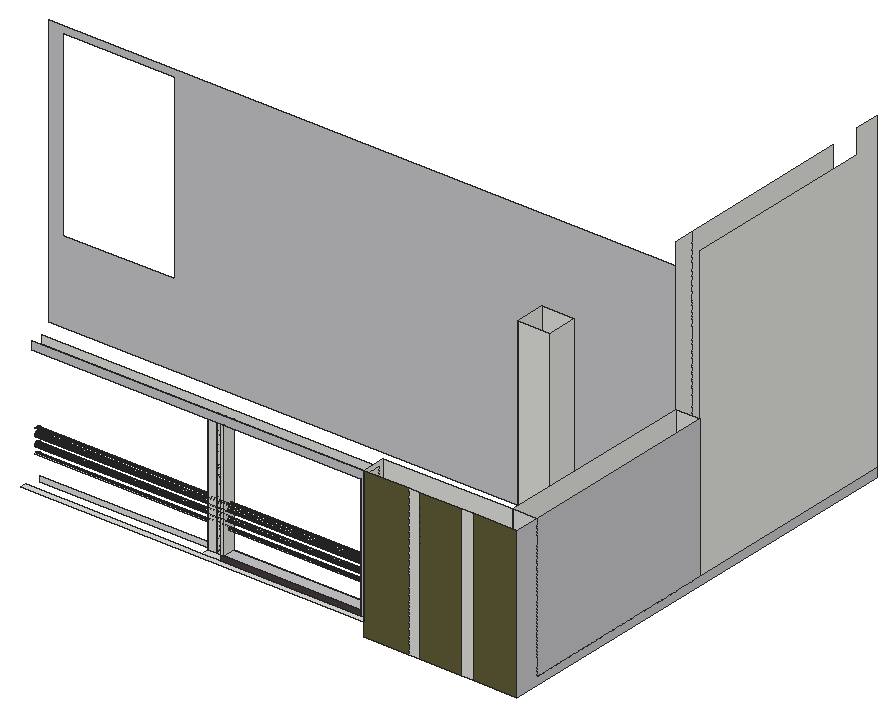
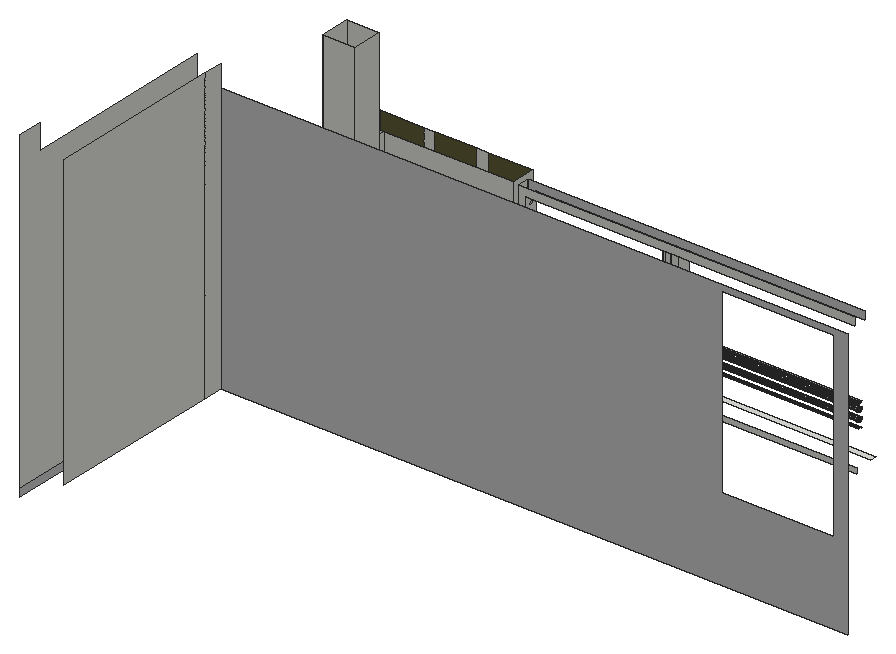
# SketchUp Ruby script. Lengths in inches.
U = 1.inch
M = Sketchup.active_model
def pt(a) = Geom::Point3d.new(a.map { |v| v * U })
def face(e, loops, mat)
  f = e.add_face(loops[0].map { |a| pt(a) })
  loops[1..].each { |l| e.add_face(l.map { |a| pt(a) }).erase! }
  f.material = f.back_material = mat if mat
  f
end
# faces: each face lists its corners as indices into pts; further lists are holes
def faces(e, pts, list, mat = nil) = list.each { |f| face(e, (f[0].is_a?(Array) ? f : [f]).map { |l| l.map { |i| pts[i] } }, mat) }
# xy, xz, yz: faces in a plane at the given z, y or x. An outline is a flat list of corners, or four numbers for a rectangle; further outlines are holes
def ring(l) = l.size == 4 ? [[l[0], l[1]], [l[2], l[1]], [l[2], l[3]], [l[0], l[3]]] : l.each_slice(2).to_a
def flat(e, list, mat, &to3) = list.each { |f| face(e, (f[0].is_a?(Array) ? f : [f]).map { |l| ring(l).map { |u, v| to3.(u, v) } }, mat) }
def xy(e, z, list, mat = nil) = flat(e, list, mat) { |x, y| [x, y, z] }
def xz(e, y, list, mat = nil) = flat(e, list, mat) { |x, z| [x, y, z] }
def yz(e, x, list, mat = nil) = flat(e, list, mat) { |y, z| [x, y, z] }
def lines(e, pts, list) = list.each { |a, b| e.add_line(pt(pts[a]), pt(pts[b])) }
# prism: a flat outline (further loops are holes) pulled along v
def prism(e, loops, v, mat = nil)
  f = face(e, loops, mat); d = Geom::Vector3d.new(v.map { |x| x * U })
  f.pushpull(f.normal.samedirection?(d) ? d.length : -d.length)
end
def box(e, o, s, mat = nil) = prism(e, [[o, [o[0] + s[0], o[1], o[2]], [o[0] + s[0], o[1] + s[1], o[2]], [o[0], o[1] + s[1], o[2]]]], [0, 0, s[2]], mat)
def at(x, y, z, deg = 0) = Geom::Transformation.translation(pt([x, y, z])) * Geom::Transformation.rotation(ORIGIN, Z_AXIS, deg.degrees)
def axes(o, x, y, z) = Geom::Transformation.new([*x, 0, *y, 0, *z, 0, *pt(o).to_a, 1])
def part(name) = M.definitions.add(name)
# library, detail: a bought-in or finely detailed component or shape, given as its bounding box
def library(name, o, s) = part(name).tap { |d| box(d.entities, o, s) }
def detail(e, o, s) = box(e.add_group.entities, o, s)
def put(e, d, t, mat = nil) = e.add_instance(d, t).tap { |i| i.material = mat if mat }
def group(e, t, mat = nil) = e.add_group.tap { |g| g.transformation = t; g.material = mat if mat }.entities
root = M.entities
M.materials.add("[0057_DarkKhaki]").color = [96, 93, 54]
M.materials.add("[Asphalt New]").color = [67, 60, 62]
M.materials.add("[Polished Concrete New]").color = [200, 200, 203]
M.materials.add("[Polished Concrete Old]").color = [229, 229, 229]
xy(root,9,[[1072.84,249.9,1099.23,472.99],[1027.11,314.12,1062.63,346.6]])
xy(root,14.9375,[[555.05,223.5,931.07,223.5,931.07,230.1,922.51,230.1,922.51,230.11,768.81,230.26,748.36,230.28,727.92,230.3,555.05,230.47],[922.51,230.1,922.51,230.11,931.07,230.1],[931.07,230.1,931.07,243.6875,922.51,243.6875,922.51,230.11],[922.51,230.11,768.81,230.26,768.82,243.84,931.07,243.6875,922.51,243.6875],[768.81,230.26,748.36,230.28,748.38,243.86,768.82,243.84]])
xy(root,21,[[754.67,230.27,754.67,243.86,764.33,243.85,764.33,230.27]])
xy(root,21,[[922.51,230.11,922.51,243.6875,931.07,243.6875,772.74,243.84,772.74,230.26]],"[Polished Concrete New]")
xz(root,223.5,[[980.52,0,992.48,163.5625],[1038.1875,0,1050.15,163.5625]])
xz(root,223.5,[[931.03,0,980.52,0,980.52,163.5625,931.07,163.5625,931.07,14.9375,931.03,14.9375],[992.48,0,1038.1875,163.5625],[1050.15,0,1099.23,163.5625]],"[0057_DarkKhaki]")
xz(root,230.1,[[922.51,14.9375,931.07,14.9375,931.07,158,562.43,158,562.43,149.47,922.51,149.47]],"[Polished Concrete New]")
xz(root,230.26,[[768.81,21,772.74,149.47],[768.81,21,772.74,149.47]])
xz(root,230.27,[[754.67,21,764.33,149.47]])
xz(root,243.6875,[[922.51,14.9375,931.07,21],[922.51,21,922.51,149.47,562.43,149.47,562.43,158.26,931.07,158.26,931.07,21]])
xz(root,249.9,[[555.05,9,931.07,14.9375],[931.07,9,1072.84,163.5625],[1072.84,9,1099.23,163.5625]])
xz(root,314.12,[[1027.11,9,1062.63,304.3125]])
xz(root,346.6,[[1027.11,9,1062.63,304.3125]])
xz(root,472.99,[[1072.84,9,1099.23,163.5625]])
xz(root,472.99,[[[386.67,9,1072.84,304.3125],[402.52,98.87,525.08,297.18]]],"[Polished Concrete New]")
yz(root,754.67,[[230.27,21,243.86,149.47]])
yz(root,764.33,[[230.27,21,243.85,149.47]])
yz(root,772.74,[[230.26,21,243.84,149.47]])
yz(root,922.51,[[[230.1,14.9375,230.1,149.47,243.6875,149.47,243.6875,21,230.11,21,230.11,14.9375],[236.62,77.51,237.7,77.65,238.71,78.07,239.58,78.74,240.24,79.6,240.66,80.61,240.81,81.7,240.66,82.78,240.24,83.79,239.58,84.66,238.71,85.32,237.7,85.74,236.62,85.89,235.53,85.74,234.52,85.32,233.66,84.66,232.99,83.79,232.57,82.78,232.43,81.7,232.57,80.61,232.99,79.6,233.66,78.74,234.52,78.07,235.53,77.65],[236.71,138.15,237.35,138.24,237.93,138.48,238.4375,138.87,238.83,139.375,239.07,139.96,239.15,140.59,239.07,141.22,238.83,141.8125,238.4375,142.32,237.93,142.7,237.35,142.95,236.71,143.03,236.08,142.95,235.5,142.7,234.99,142.32,234.6,141.8125,234.36,141.22,234.28,140.59,234.36,139.96,234.6,139.375,234.99,138.87,235.5,138.48,236.08,138.24],[236.71,89.28,237.35,89.36,237.93,89.61,238.4375,89.99,238.83,90.5,239.07,91.09,239.15,91.72,239.07,92.35,238.83,92.9375,238.4375,93.44,237.93,93.83,237.35,94.07,236.71,94.15,236.08,94.07,235.5,93.83,234.99,93.44,234.6,92.9375,234.36,92.35,234.28,91.72,234.36,91.09,234.6,90.5,234.99,89.99,235.5,89.61,236.08,89.36],[236.71,129.34,237.35,129.43,237.93,129.67,238.4375,130.06,238.83,130.5625,239.07,131.15,239.15,131.78,239.07,132.41,238.83,133,238.4375,133.5,237.93,133.89,237.35,134.13,236.71,134.22,236.08,134.13,235.5,133.89,234.99,133.5,234.6,133,234.36,132.41,234.28,131.78,234.36,131.15,234.6,130.5625,234.99,130.06,235.5,129.67,236.08,129.43],[236.71,98.28,237.35,98.36,237.93,98.61,238.4375,98.99,238.83,99.5,239.07,100.09,239.15,100.72,239.07,101.35,238.83,101.9375,238.4375,102.44,237.93,102.83,237.35,103.07,236.71,103.15,236.08,103.07,235.5,102.83,234.99,102.44,234.6,101.9375,234.36,101.35,234.28,100.72,234.36,100.09,234.6,99.5,234.99,98.99,235.5,98.61,236.08,98.36],[236.71,118.53,237.35,118.61,237.93,118.86,238.4375,119.24,238.83,119.75,239.07,120.34,239.15,120.97,239.07,121.6,238.83,122.1875,238.4375,122.69,237.93,123.08,237.35,123.32,236.71,123.4,236.08,123.32,235.5,123.08,234.99,122.69,234.6,122.1875,234.36,121.6,234.28,120.97,234.36,120.34,234.6,119.75,234.99,119.24,235.5,118.86,236.08,118.61],[236.71,108.15,237.35,108.24,237.93,108.48,238.4375,108.87,238.83,109.375,239.07,109.96,239.15,110.59,239.07,111.22,238.83,111.8125,238.4375,112.32,237.93,112.7,237.35,112.95,236.71,113.03,236.08,112.95,235.5,112.7,234.99,112.32,234.6,111.8125,234.36,111.22,234.28,110.59,234.36,109.96,234.6,109.375,234.99,108.87,235.5,108.48,236.08,108.24],[236.71,23.9,237.35,23.99,237.93,24.23,238.4375,24.62,238.83,25.125,239.07,25.71,239.15,26.34,239.07,26.97,238.83,27.5625,238.4375,28.07,237.93,28.45,237.35,28.7,236.71,28.78,236.08,28.7,235.5,28.45,234.99,28.07,234.6,27.5625,234.36,26.97,234.28,26.34,234.36,25.71,234.6,25.125,234.99,24.62,235.5,24.23,236.08,23.99],[236.71,70.22,237.35,70.3,237.93,70.54,238.4375,70.93,238.83,71.4375,239.07,72.02,239.15,72.65,239.07,73.29,238.83,73.875,238.4375,74.38,237.93,74.77,237.35,75.01,236.71,75.09,236.08,75.01,235.5,74.77,234.99,74.38,234.6,73.875,234.36,73.29,234.28,72.65,234.36,72.02,234.6,71.4375,234.99,70.93,235.5,70.54,236.08,70.3],[236.71,33.4,237.35,33.49,237.93,33.73,238.4375,34.12,238.83,34.625,239.07,35.21,239.15,35.84,239.07,36.47,238.83,37.0625,238.4375,37.57,237.93,37.95,237.35,38.2,236.71,38.28,236.08,38.2,235.5,37.95,234.99,37.57,234.6,37.0625,234.36,36.47,234.28,35.84,234.36,35.21,234.6,34.625,234.99,34.12,235.5,33.73,236.08,33.49],[236.71,61.84,237.35,61.93,237.93,62.17,238.4375,62.56,238.83,63.0625,239.07,63.65,239.15,64.28,239.07,64.91,238.83,65.5,238.4375,66,237.93,66.39,237.35,66.63,236.71,66.72,236.08,66.63,235.5,66.39,234.99,66,234.6,65.5,234.36,64.91,234.28,64.28,234.36,63.65,234.6,63.0625,234.99,62.56,235.5,62.17,236.08,61.93],[236.71,41.84,237.35,41.93,237.93,42.17,238.4375,42.56,238.83,43.0625,239.07,43.65,239.15,44.28,239.07,44.91,238.83,45.5,238.4375,46,237.93,46.39,237.35,46.63,236.71,46.72,236.08,46.63,235.5,46.39,234.99,46,234.6,45.5,234.36,44.91,234.28,44.28,234.36,43.65,234.6,43.0625,234.99,42.56,235.5,42.17,236.08,41.93],[236.71,52.03,237.35,52.11,237.93,52.36,238.4375,52.74,238.83,53.25,239.07,53.84,239.15,54.47,239.07,55.1,238.83,55.6875,238.4375,56.19,237.93,56.58,237.35,56.82,236.71,56.9,236.08,56.82,235.5,56.58,234.99,56.19,234.6,55.6875,234.36,55.1,234.28,54.47,234.36,53.84,234.6,53.25,234.99,52.74,235.5,52.36,236.08,52.11]],[230.11,14.9375,243.6875,21],[236.71,23.9,237.35,23.99,237.93,24.23,238.4375,24.62,238.83,25.125,239.07,25.71,239.15,26.34,239.07,26.97,238.83,27.5625,238.4375,28.07,237.93,28.45,237.35,28.7,236.71,28.78,236.08,28.7,235.5,28.45,234.99,28.07,234.6,27.5625,234.36,26.97,234.28,26.34,234.36,25.71,234.6,25.125,234.99,24.62,235.5,24.23,236.08,23.99],[236.71,33.4,237.35,33.49,237.93,33.73,238.4375,34.12,238.83,34.625,239.07,35.21,239.15,35.84,239.07,36.47,238.83,37.0625,238.4375,37.57,237.93,37.95,237.35,38.2,236.71,38.28,236.08,38.2,235.5,37.95,234.99,37.57,234.6,37.0625,234.36,36.47,234.28,35.84,234.36,35.21,234.6,34.625,234.99,34.12,235.5,33.73,236.08,33.49],[236.71,41.84,237.35,41.93,237.93,42.17,238.4375,42.56,238.83,43.0625,239.07,43.65,239.15,44.28,239.07,44.91,238.83,45.5,238.4375,46,237.93,46.39,237.35,46.63,236.71,46.72,236.08,46.63,235.5,46.39,234.99,46,234.6,45.5,234.36,44.91,234.28,44.28,234.36,43.65,234.6,43.0625,234.99,42.56,235.5,42.17,236.08,41.93],
  [236.71,52.03,237.35,52.11,237.93,52.36,238.4375,52.74,238.83,53.25,239.07,53.84,239.15,54.47,239.07,55.1,238.83,55.6875,238.4375,56.19,237.93,56.58,237.35,56.82,236.71,56.9,236.08,56.82,235.5,56.58,234.99,56.19,234.6,55.6875,234.36,55.1,234.28,54.47,234.36,53.84,234.6,53.25,234.99,52.74,235.5,52.36,236.08,52.11],[236.71,61.84,237.35,61.93,237.93,62.17,238.4375,62.56,238.83,63.0625,239.07,63.65,239.15,64.28,239.07,64.91,238.83,65.5,238.4375,66,237.93,66.39,237.35,66.63,236.71,66.72,236.08,66.63,235.5,66.39,234.99,66,234.6,65.5,234.36,64.91,234.28,64.28,234.36,63.65,234.6,63.0625,234.99,62.56,235.5,62.17,236.08,61.93],[236.71,70.22,237.35,70.3,237.93,70.54,238.4375,70.93,238.83,71.4375,239.07,72.02,239.15,72.65,239.07,73.29,238.83,73.875,238.4375,74.38,237.93,74.77,237.35,75.01,236.71,75.09,236.08,75.01,235.5,74.77,234.99,74.38,234.6,73.875,234.36,73.29,234.28,72.65,234.36,72.02,234.6,71.4375,234.99,70.93,235.5,70.54,236.08,70.3]])
yz(root,931.07,[[223.5,14.9375,223.5,163.5625,249.9,163.5625,249.9,14.9375,243.6875,14.9375,243.6875,158.26,230.1,158.26,230.1,14.9375],[230.1,14.9375,243.6875,158.26]])
yz(root,1027.11,[[314.12,9,346.6,304.3125]])
yz(root,1062.63,[[314.12,9,346.6,304.3125]])
yz(root,1072.84,[[249.9,9,472.99,163.5625],[472.99,9,494.96,328.125],[494.96,9,688.57,328.125]])
yz(root,1099.23,[[472.99,9,714.96,9,714.96,354.875,688.57,354.875,688.57,328.125,472.99,328.125]])
yz(root,1099.23,[[223.5,0,714.96,0,714.96,9,249.9,9,249.9,163.5625,223.5,163.5625],[249.9,9,472.99,163.5625]],"[Polished Concrete New]")
p = [[922.51,230.11,21],[772.74,230.26,21],[768.81,230.26,21],[768.81,230.26,14.9375],[922.51,230.11,14.9375],[931.07,243.6875,14.9375],
  [768.82,243.84,14.9375],[768.82,243.84,149.47],[772.74,243.84,149.47],[772.74,243.84,21],[931.07,243.6875,21],[748.38,243.86,14.9375],
  [748.38,243.86,21],[754.67,243.86,21],[764.33,243.85,21],[764.33,243.85,149.47],[764.33,230.27,149.47],[764.33,230.27,21],
  [768.81,230.26,149.47],[754.67,243.86,149.47],[922.51,234.6,45.5],[922.51,234.99,46],[562.43,234.99,46],[562.43,234.6,45.5],
  [922.51,235.5,46.39],[562.43,235.5,46.39],[922.51,237.93,46.39],[922.51,238.4375,46],[562.43,238.4375,46],[562.43,237.93,46.39],
  [922.51,236.08,46.63],[562.43,236.08,46.63],[922.51,237.35,46.63],[562.43,237.35,46.63],[922.51,236.71,46.72],[562.43,236.71,46.72],
  [922.51,236.71,52.03],[922.51,236.08,52.11],[562.43,236.08,52.11],[562.43,236.71,52.03],[922.51,237.35,52.11],[562.43,237.35,52.11],
  [922.51,235.5,52.36],[562.43,235.5,52.36],[922.51,237.93,52.36],[562.43,237.93,52.36],[922.51,234.99,52.74],[562.43,234.99,52.74],
  [922.51,238.4375,52.74],[562.43,238.4375,52.74],[922.51,234.6,53.25],[562.43,234.6,53.25],[922.51,238.83,53.25],[562.43,238.83,53.25],
  [922.51,234.36,53.84],[562.43,234.36,53.84],[922.51,239.07,53.84],[562.43,239.07,53.84],[922.51,234.28,54.47],[562.43,234.28,54.47],
  [922.51,239.15,54.47],[562.43,239.15,54.47],[922.51,234.36,55.1],[562.43,234.36,55.1],[922.51,239.07,55.1],[562.43,239.07,55.1],
  [922.51,234.6,55.6875],[562.43,234.6,55.6875],[922.51,238.83,55.6875],[562.43,238.83,55.6875],[922.51,234.99,56.19],[562.43,234.99,56.19],
  [922.51,238.4375,56.19],[562.43,238.4375,56.19],[922.51,235.5,56.58],[562.43,235.5,56.58],[922.51,237.93,56.58],[562.43,237.93,56.58],
  [922.51,236.08,56.82],[562.43,236.08,56.82],[922.51,237.35,56.82],[562.43,237.35,56.82],[922.51,236.71,56.9],[562.43,236.71,56.9],
  [922.51,236.71,61.84],[922.51,236.08,61.93],[562.43,236.08,61.93],[562.43,236.71,61.84],[922.51,237.35,61.93],[562.43,237.35,61.93],
  [922.51,235.5,62.17],[562.43,235.5,62.17],[922.51,237.93,62.17],[562.43,237.93,62.17],[922.51,234.99,62.56],[562.43,234.99,62.56],
  [922.51,238.4375,62.56],[562.43,238.4375,62.56],[922.51,234.6,63.0625],[562.43,234.6,63.0625],[922.51,238.83,63.0625],[562.43,238.83,63.0625],
  [922.51,234.36,63.65],[562.43,234.36,63.65],[922.51,239.07,63.65],[562.43,239.07,63.65],[922.51,234.28,64.28],[562.43,234.28,64.28],
  [922.51,239.15,64.28],[562.43,239.15,64.28],[922.51,234.36,64.91],[562.43,234.36,64.91],[922.51,239.07,64.91],[562.43,239.07,64.91],
  [922.51,234.6,65.5],[562.43,234.6,65.5],[922.51,238.83,65.5],[562.43,238.83,65.5],[922.51,234.99,66],[562.43,234.99,66],
  [922.51,238.4375,66],[562.43,238.4375,66],[922.51,235.5,66.39],[562.43,235.5,66.39],[922.51,237.93,66.39],[562.43,237.93,66.39],
  [922.51,236.08,66.63],[562.43,236.08,66.63],[922.51,237.35,66.63],[562.43,237.35,66.63],[922.51,236.71,66.72],[562.43,236.71,66.72],
  [922.51,236.71,70.22],[922.51,236.08,70.3],[562.43,236.08,70.3],[562.43,236.71,70.22],[922.51,237.35,70.3],[562.43,237.35,70.3],
  [922.51,235.5,70.54],[562.43,235.5,70.54],[922.51,237.93,70.54],[562.43,237.93,70.54],[922.51,234.99,70.93],[562.43,234.99,70.93],
  [922.51,238.4375,70.93],[562.43,238.4375,70.93],[922.51,234.6,71.4375],[562.43,234.6,71.4375],[922.51,238.83,71.4375],[562.43,238.83,71.4375],
  [931.03,223.5,15.46],[931.03,223.5,14.9375]]
faces(root,p,[[0,1,2,3,4]],"[Asphalt New]")
faces(root,p,[[1,2,3,4,0],[5,6,7,8,9,10],[6,11,12,13,14,15,7],[16,17,2,18],[17,2,18,16],[14,13,19,15]])
faces(root,p,[[20,21,22,23],[21,24,25,22],[26,27,28,29],[24,30,31,25],[32,26,29,33],[30,34,35,31],[34,32,33,35],[36,37,38,39],
  [40,36,39,41],[37,42,43,38],[44,40,41,45],[42,46,47,43],[48,44,45,49],[46,50,51,47],[52,48,49,53],[50,54,55,51],
  [56,52,53,57],[54,58,59,55],[60,56,57,61],[58,62,63,59],[64,60,61,65],[62,66,67,63],[68,64,65,69],[66,70,71,67],
  [72,68,69,73],[70,74,75,71],[76,72,73,77],[74,78,79,75],[80,76,77,81],[78,82,83,79],[82,80,81,83],[84,85,86,87],
  [88,84,87,89],[85,90,91,86],[92,88,89,93],[90,94,95,91],[96,92,93,97],[94,98,99,95],[100,96,97,101],[98,102,103,99],
  [104,100,101,105],[102,106,107,103],[108,104,105,109],[106,110,111,107],[112,108,109,113],[110,114,115,111],[116,112,113,117],[114,118,119,115],
  [120,116,117,121],[118,122,123,119],[124,120,121,125],[122,126,127,123],[128,124,125,129],[126,130,131,127],[130,128,129,131],[132,133,134,135],
  [136,132,135,137],[133,138,139,134],[140,136,137,141],[138,142,143,139],[144,140,141,145],[142,146,147,143],[148,144,145,149]],"[Polished Concrete Old]")
lines(root,p,[[150,151]])
